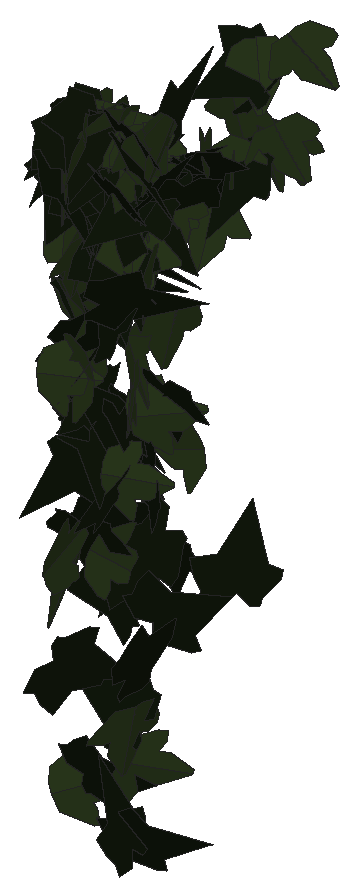
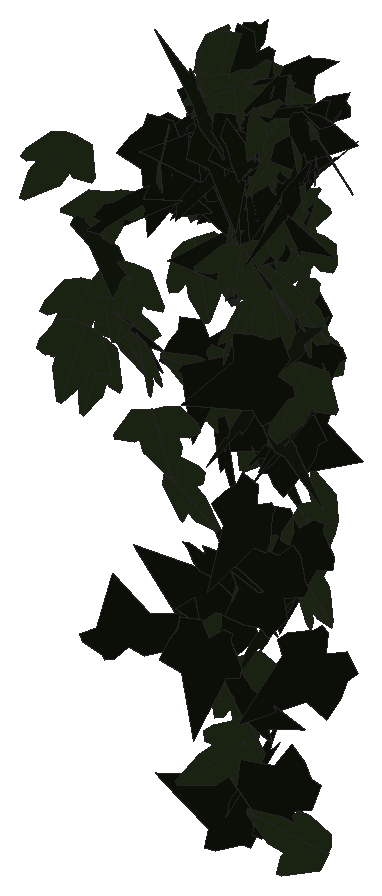
# SketchUp Ruby script. Lengths in inches.
U = 1.inch
M = Sketchup.active_model
def pt(a) = Geom::Point3d.new(a.map { |v| v * U })
def face(e, loops, mat)
  f = e.add_face(loops[0].map { |a| pt(a) })
  loops[1..].each { |l| e.add_face(l.map { |a| pt(a) }).erase! }
  f.material = f.back_material = mat if mat
  f
end
# faces: each face lists its corners as indices into pts; further lists are holes
def faces(e, pts, list, mat = nil) = list.each { |f| face(e, (f[0].is_a?(Array) ? f : [f]).map { |l| l.map { |i| pts[i] } }, mat) }
# xy, xz, yz: faces in a plane at the given z, y or x. An outline is a flat list of corners, or four numbers for a rectangle; further outlines are holes
def ring(l) = l.size == 4 ? [[l[0], l[1]], [l[2], l[1]], [l[2], l[3]], [l[0], l[3]]] : l.each_slice(2).to_a
def flat(e, list, mat, &to3) = list.each { |f| face(e, (f[0].is_a?(Array) ? f : [f]).map { |l| ring(l).map { |u, v| to3.(u, v) } }, mat) }
def xy(e, z, list, mat = nil) = flat(e, list, mat) { |x, y| [x, y, z] }
def xz(e, y, list, mat = nil) = flat(e, list, mat) { |x, z| [x, y, z] }
def yz(e, x, list, mat = nil) = flat(e, list, mat) { |y, z| [x, y, z] }
def lines(e, pts, list) = list.each { |a, b| e.add_line(pt(pts[a]), pt(pts[b])) }
# prism: a flat outline (further loops are holes) pulled along v
def prism(e, loops, v, mat = nil)
  f = face(e, loops, mat); d = Geom::Vector3d.new(v.map { |x| x * U })
  f.pushpull(f.normal.samedirection?(d) ? d.length : -d.length)
end
def box(e, o, s, mat = nil) = prism(e, [[o, [o[0] + s[0], o[1], o[2]], [o[0] + s[0], o[1] + s[1], o[2]], [o[0], o[1] + s[1], o[2]]]], [0, 0, s[2]], mat)
def at(x, y, z, deg = 0) = Geom::Transformation.translation(pt([x, y, z])) * Geom::Transformation.rotation(ORIGIN, Z_AXIS, deg.degrees)
def axes(o, x, y, z) = Geom::Transformation.new([*x, 0, *y, 0, *z, 0, *pt(o).to_a, 1])
def part(name) = M.definitions.add(name)
# library, detail: a bought-in or finely detailed component or shape, given as its bounding box
def library(name, o, s) = part(name).tap { |d| box(d.entities, o, s) }
def detail(e, o, s) = box(e.add_group.entities, o, s)
def put(e, d, t, mat = nil) = e.add_instance(d, t).tap { |i| i.material = mat if mat }
def group(e, t, mat = nil) = e.add_group.tap { |g| g.transformation = t; g.material = mat if mat }.entities
root = M.entities
M.materials.add("efeu1").color = [18, 25, 13]
M.materials.add("efeu2").color = [43, 57, 29]
c1 = part("ivyleaf_9")
p = [[1.54,2.16,1.25],[1.36,2.04,1.19],[-0.21,0.99,0.68],[-0.71,1.11,0.82],[-0.85,0.86,0.67],[-0.8,0.17,0.21],
  [-0.9,-0.01,0.1],[-0.67,-0.16,-0.02],[-0.08,-0.08,-0.05],[-0.03,-0.6,-0.4],[0.65,-0.88,-0.66],[0.83,-0.6,-0.49],
  [1.29,-0.42,-0.43],[1.8125,-0.07,-0.26],[1.21,0.44,0.15]]
faces(c1.entities,p,[[0,1,2,3,4,5,6,7,8,9,10,11,12,13,14]],"efeu1")
c2 = part("ivyleaf_10")
p = [[0,0.5,-0.03],[-0.0625,2.02,-0.43],[-0.19,2.01,-0.46],[-0.54,1.05,-0.29],[-0.52,0.625,-0.18],[-0.83,0.76,-0.28],
  [-1.16,0.64,-0.33],[-1.15,0.33,-0.24],[-0.77,-0.39,0.02],[-0.3,-0.51,0.16],[0.04,-0.48,0.23],[-0.02,2.01,-0.4375],
  [-0.06,2.01,-0.43],[0.04,-0.49,0.23],[0.67,-0.49,0.14],[1.38,0.36,-0.2],[1.375,0.51,-0.24],[0.81,0.65,-0.19],
  [0.62,0.59,-0.15],[0.6,1.09,-0.28],[0.5,1.23,-0.31]]
faces(c2.entities,p,[[0,1,2,3,4,5,6,7,8,9,10],[11,12,0,13,14,15,16,17,18,19,20]],"efeu2")
put(root,c1,axes([545.61,136.74,199.4],[0.63239,0.17677,0.4577],[0.42669,0.17049,-0.65539],[-0.24223,0.7618,0.04047]))
put(root,c2,axes([546.11,140.69,199.7],[0.68213,0.44243,-0.14411],[-0.17077,0.00015,-0.80787],[-0.43284,0.69719,0.09162]))
put(root,c1,axes([546.1,134.98,203.92],[0.41864,-0.09963,-0.78482],[-0.51595,0.63873,-0.3563],[0.59972,0.61905,0.24132]))
put(root,c2,axes([546.69,134.25,199.875],[0.06447,0.00912,-0.85901],[-0.63743,0.57799,-0.0417],[0.5759,0.63873,0.05001]))
put(root,c2,axes([546.13,134.99,198.29],[-0.41829,-0.63523,-0.40609],[0.26002,0.31436,-0.75958],[0.70768,-0.49097,0.03906]))
put(root,c2,axes([546.22,135.08,204.94],[0.42247,-0.7153,-0.04041],[0.04281,0.07203,-0.82749],[0.71516,0.41824,0.0734]))
put(root,c1,axes([545.76,135.46,199.64],[0.53861,-0.60321,-0.07073],[0.1239,0.20168,-0.77649],[0.59457,0.50441,0.22588]))
put(root,c1,axes([546.33,135.1,205.17],[0.02686,-0.08138,-0.82508],[0.27504,-0.77789,0.08568],[-0.78214,-0.27634,0.0018]))
put(root,c1,axes([546.68,134.18,205.14],[-0.76345,0.21406,-0.26205],[0.25896,-0.04664,-0.79254],[-0.21779,-0.80582,-0.02374]))
put(root,c1,axes([546.89,135.11,196.85],[-0.59699,0.5547,0.02639],[-0.02109,0.01607,-0.81491],[-0.55492,-0.59736,0.00258]))
put(root,c1,axes([547.1875,134.78,202.4],[-0.38586,0.27044,0.67565],[-0.52247,0.42944,-0.47026],[-0.50664,-0.64883,-0.02962]))
put(root,c2,axes([546.625,135.43,200.49],[-0.11591,-0.80635,0.00121],[0.0201,-0.00411,-0.81438],[0.8061,-0.11584,0.02048]))
put(root,c2,axes([546.48,135.21,205.03],[0.02633,-0.46906,-0.67824],[0.19734,0.66245,-0.45048],[0.80067,-0.14785,0.13334]))
put(root,c2,axes([546.66,135.04,202.78],[-0.10519,-0.61205,0.52001],[0.05814,-0.52888,-0.61073],[0.80103,-0.04199,0.11261]))
put(root,c1,axes([546.4,134.43,203.5625],[-0.20295,-0.72127,0.44661],[0.10126,-0.47653,-0.72356],[0.84228,-0.1165,0.1946]))
put(root,c2,axes([546.58,134.14,192.11],[0.23697,-0.69809,0.4273],[0.16665,-0.39438,-0.73672],[0.80134,0.28845,0.02686]))
put(root,c2,axes([546.32,134.5,201.97],[0.64893,0.30322,0.3824],[0.30225,0.24981,-0.711],[-0.38316,0.71059,0.08678]))
put(root,c1,axes([546.46,133.89,198.91],[0.4772,0.52153,0.62438],[0.41266,0.46866,-0.70685],[-0.70111,0.63082,0.00894]))
put(root,c2,axes([546.17,134.57,185.02],[0.32928,0.01072,-0.79971],[0.79309,0.10729,0.32799],[0.10327,-0.85817,0.03102]))
put(root,c1,axes([546.23,135.67,192.52],[0.70579,0.31997,-0.30043],[0.21253,0.24863,0.76407],[0.38402,-0.72566,0.12931]))
put(root,c1,axes([546.9,134.19,193.42],[0.65453,0.36972,-0.41326],[-0.35074,-0.21914,-0.75156],[-0.42949,0.74241,-0.01604]))
put(root,c1,axes([546.54,135.07,196.45],[0.17609,-0.79948,0.16462],[0.02458,-0.16314,-0.81857],[0.81588,0.17746,-0.01087]))
put(root,c1,axes([546.71,136.125,195.03],[0.77795,0.04309,-0.26893],[-0.26975,0.00954,-0.77879],[-0.0376,0.82306,0.0231]))
put(root,c2,axes([546.71,140.51,201.54],[0.67204,-0.44105,0.22768],[0.20511,-0.10222,-0.80342],[0.45199,0.70216,0.02606]))
put(root,c1,axes([546.89,135.14,205.49],[-0.53508,-0.61574,-0.12557],[0.09523,0.08357,-0.81557],[0.62115,-0.54323,0.01686]))
put(root,c2,axes([546.74,133.73,204.45],[-0.41519,0.41173,-0.57655],[0.18834,-0.58007,-0.54987],[-0.68298,-0.41026,0.19885]))
put(root,c2,axes([547.03,135.24,205.375],[-0.06291,-0.81765,-0.05684],[-0.01553,0.05818,-0.81982],[0.81947,-0.06167,-0.0199]))
put(root,c1,axes([546.61,134.11,205.38],[0.03815,-0.75855,-0.42726],[0.08293,0.42889,-0.75404],[0.86664,-0.00765,0.09097]))
put(root,c2,axes([546.86,135.02,205.39],[0.76183,0.29375,-0.05461],[-0.04328,-0.03951,-0.81622],[-0.29563,0.76276,-0.02125]))
put(root,c2,axes([546.89,135.35,200.86],[-0.19322,-0.5596,-0.56445],[0.22203,0.51977,-0.5913],[0.76319,-0.29289,0.02912]))
put(root,c2,axes([546.98,141.9,201.81],[-0.80811,0.1931,-0.06685],[0.06148,-0.03029,-0.83072],[-0.19487,-0.8103,0.01512]))
put(root,c1,axes([546.8,133.32,189.59],[0.02204,0.08481,-0.91651],[-0.16467,0.90235,0.07954],[0.90558,0.16201,0.03677]))
put(root,c2,axes([547.07,140.625,203.3],[-0.80095,-0.1323,-0.04872],[0.05105,-0.01019,-0.81159],[0.13142,-0.80236,0.01834]))
put(root,c2,axes([547.6,133.39,198.49],[0.21564,-0.19118,-0.90246],[-0.69715,0.57316,-0.288],[0.60412,0.72967,-0.01023]))
put(root,c1,axes([546.6,133.5,204.46],[0.50245,-0.71675,-0.00209],[-0.00204,0.00112,-0.87532],[0.71675,0.50246,-0.00103]))
put(root,c1,axes([547.08,134.77,204.45],[0.6357,0.37801,-0.34333],[-0.35969,-0.05768,-0.72951],[-0.36248,0.72019,0.12178]))
put(root,c1,axes([547.21,134.02,195.8125],[-0.02693,-0.00723,-0.85682],[0.23533,-0.82434,-0.00044],[-0.8239,-0.23522,0.02788]))
put(root,c1,axes([547.18,137.35,191.61],[0.63912,0.27311,-0.45217],[-0.40769,-0.1963,-0.69482],[-0.33591,0.75789,-0.01703]))
put(root,c2,axes([547.2,133.8,202.13],[0.06647,-0.85038,-0.03459],[0.00194,0.03485,-0.85296],[0.85108,0.06633,0.00464]))
put(root,c2,axes([547.24,132.76,192.94],[0.16811,-0.30744,0.92992],[-0.32559,0.87232,0.34726],[-0.92372,-0.36342,0.04684]))
put(root,c1,axes([546.94,135.54,190.92],[0.54706,-0.68574,-0.42646],[0.26362,-0.33523,0.87721],[-0.76329,-0.60726,-0.00268]))
put(root,c1,axes([547.55,135.07,201.36],[-0.71082,0.40271,-0.09212],[0.08434,-0.03801,-0.81693],[-0.40441,-0.71576,-0.00845]))
put(root,c2,axes([546.58,133.37,198.25],[0.13669,-0.19673,-0.77637],[0.78336,-0.1311,0.17114],[-0.16671,-0.77733,0.16762]))
put(root,c1,axes([546.97,134.5,203.62],[0.04386,-0.85651,-0.16835],[-0.02143,0.16746,-0.85754],[0.87263,0.04716,-0.0126]))
put(root,c1,axes([547.4375,133.27,198.36],[0.12962,0.51972,0.62303],[-0.01566,0.63241,-0.52429],[-0.81119,0.07084,0.10967]))
put(root,c1,axes([547.03,134.62,196.34],[0.07655,-0.80206,0.06377],[0.02846,-0.06132,-0.8054],[0.80409,0.07853,0.02243]))
put(root,c2,axes([547.48,140.42,201.96],[0.78404,-0.04348,-0.28572],[-0.28551,0.01153,-0.78524],[0.0448,0.8344,-0.00403]))
put(root,c1,axes([546.85,134.44,196.92],[-0.12305,-0.06856,-0.87052],[0.68325,0.53988,-0.1391],[0.54377,-0.69388,-0.02221]))
put(root,c2,axes([547.48,134.78,204.21],[0.04292,-0.81362,0.15034],[0.00143,-0.15047,-0.81472],[0.82739,0.04247,-0.00639]))
put(root,c1,axes([547.07,134.44,204.04],[0.36162,-0.55029,-0.57723],[-0.09742,0.59857,-0.63166],[0.79153,0.32508,0.18597]))
put(root,c2,axes([547.27,135.95,201.91],[0.40906,0.69555,0.05472],[0.02898,0.04644,-0.80692],[-0.69709,0.41008,-0.00143]))
put(root,c1,axes([547.5,134.75,204.91],[-0.39146,-0.6806,0.22902],[-0.12295,-0.19347,-0.78509],[0.7075,-0.4102,-0.00971]))
put(root,c1,axes([547.89,140.57,204.09],[-0.07567,0.62355,0.52426],[-0.27553,0.47589,-0.60579],[-0.76664,-0.23258,0.16598]))
put(root,c1,axes([547.6,140.49,201.95],[-0.77482,-0.18215,-0.25497],[0.27034,-0.04472,-0.78959],[0.15844,-0.81447,0.10037]))
put(root,c1,axes([546.9,134.83,202.18],[0.22154,-0.01211,0.8427],[0.82646,0.17379,-0.21478],[-0.16508,0.85383,0.05566]))
put(root,c2,axes([547.56,133.4,205.55],[0.21084,-0.7276,-0.46431],[-0.00285,0.47738,-0.74936],[0.86312,0.17931,0.11094]))
put(root,c2,axes([547.52,142.05,202.07],[-0.82513,-0.071,-0.10658],[0.10721,-0.00285,-0.82809],[0.07005,-0.83198,0.01193]))
put(root,c1,axes([547.6,135.31,204.32],[0.33624,0.21352,0.71521],[-0.59527,-0.39652,0.39823],[0.45028,-0.68363,-0.0076]))
put(root,c1,axes([547.72,140.73,204.82],[-0.42701,-0.41233,0.56307],[-0.31397,-0.47604,-0.5867],[0.62329,-0.52228,0.09022]))
put(root,c2,axes([547.3125,135.17,200.45],[0.78736,-0.09526,0.19053],[0.18664,-0.04317,-0.79286],[0.10268,0.80894,-0.01987]))
put(root,c1,axes([547.5,134.11,206],[-0.33067,-0.77131,0.05423],[-0.01346,-0.05323,-0.83916],[0.77309,-0.33083,0.00859]))
put(root,c2,axes([547.49,134.37,192.5625],[0.06112,0.52183,0.68495],[0.00049,0.68665,-0.52317],[-0.86108,0.03744,0.04832]))
put(root,c1,axes([546.91,134.43,185.76],[0.26983,-0.16319,0.8108],[0.71268,-0.38687,-0.31505],[0.41965,0.76193,0.01369]))
put(root,c1,axes([547.875,135.19,204.97],[-0.48149,0.44735,-0.49059],[0.2867,-0.4065,-0.65207],[-0.59883,-0.55431,0.08227]))
put(root,c2,axes([547.84,134.59,205.82],[-0.11987,-0.82428,0.1953],[-0.05748,-0.18887,-0.83245],[0.84515,-0.12975,-0.02892]))
put(root,c2,axes([548.29,136.02,190.43],[-0.20039,0.20317,-0.7828],[-0.61998,0.47927,0.2831],[0.51931,0.65057,0.03591]))
put(root,c2,axes([547.85,135.23,201.97],[0.09469,-0.76625,-0.28768],[0.00917,0.29058,-0.77094],[0.81842,0.0854,0.04192]))
put(root,c2,axes([547.35,135.35,203.32],[0.10686,-0.09981,0.80268],[0.68224,-0.42383,-0.14352],[0.43453,0.68999,0.02795]))
put(root,c2,axes([547.84,135.21,201.83],[-0.24546,0.78445,0.04881],[-0.0027,0.05029,-0.82187],[-0.78596,-0.24516,-0.01242]))
put(root,c2,axes([547.78,140.51,205.2],[0.56827,0.58383,0.07739],[0.05556,0.05393,-0.81473],[-0.58631,0.57097,-0.00219]))
put(root,c1,axes([548.3125,135.86,192.92],[-0.97657,-0.05472,-0.15829],[0.15803,0.00906,-0.9781],[0.05547,-0.98928,-0.00021]))
put(root,c1,axes([548.73,134.24,188.14],[-0.34865,0.2625,0.75661],[-0.60627,0.45266,-0.43642],[-0.52327,-0.69937,0.00152]))
put(root,c1,axes([548.35,135.25,204.51],[-0.133,0.81127,0.00535],[-0.00568,0.00449,-0.82208],[-0.81127,-0.13303,0.00488]))
put(root,c1,axes([547.78,134.56,197.13],[0.61895,-0.39521,-0.35068],[-0.24125,0.26914,-0.72913],[0.47007,0.65852,0.08754]))
put(root,c1,axes([547.4375,135.27,201.5],[0.65204,-0.24081,0.43804],[0.44754,-0.03946,-0.68788],[0.22266,0.78453,0.09986]))
put(root,c2,axes([548.1,134.84,205.54],[0.52459,0.6027,-0.26902],[-0.17902,-0.20082,-0.79902],[-0.63527,0.55429,0.00302]))
put(root,c1,axes([548.56,133.57,195.33],[-0.61045,0.56333,-0.07607],[0.05617,-0.05129,-0.83065],[-0.56566,-0.61303,-0.0004]))
put(root,c2,axes([548.71,136.6,195.28],[0.33121,-0.14022,-0.75629],[-0.67444,0.34297,-0.35895],[0.36983,0.75104,0.02271]))
put(root,c1,axes([548.06,134.34,203.26],[0.45689,0.44228,0.51735],[0.28828,0.43871,-0.62964],[-0.61657,0.53286,0.08898]))
put(root,c2,axes([548.15,141.04,202.65],[-0.46181,-0.62071,-0.33517],[0.3329,0.16142,-0.75763],[0.62193,-0.54731,0.15666]))
put(root,c1,axes([547.73,134.29,201.73],[0.31058,-0.53856,0.66865],[0.53052,-0.43869,-0.59975],[0.67505,0.59254,0.16371]))
put(root,c1,axes([548.42,134.42,202.39],[-0.29731,-0.57673,0.50695],[-0.06399,-0.52312,-0.63265],[0.76519,-0.26783,0.14406]))
put(root,c1,axes([549.04,134.79,203.65],[-0.37806,0.79541,0.46608],[-0.18486,0.42811,-0.88056],[-0.90318,-0.42058,-0.01487]))
put(root,c1,axes([548.44,135.27,204.59],[0.68503,0.42401,-0.16594],[-0.22759,0.05921,-0.78822],[-0.39437,0.70235,0.16663]))
put(root,c1,axes([549.04,133.05,200.46],[-0.25009,0.51858,0.59693],[-0.27243,0.53123,-0.57564],[-0.74231,-0.36968,0.01015]))
put(root,c2,axes([548.52,134.4,199.19],[-0.32648,0.79351,0.09053],[-0.04173,0.08072,-0.85801],[-0.79757,-0.32905,0.00783]))
put(root,c2,axes([548.48,134.6,205.35],[0.48386,0.66196,-0.08873],[-0.07735,-0.05329,-0.81936],[-0.66338,0.48903,0.03082]))
put(root,c1,axes([548.32,133.89,202.45],[-0.48763,-0.47094,-0.5863],[0.46477,0.36061,-0.67621],[0.5912,-0.67193,0.04801]))
put(root,c1,axes([548.48,133.32,204.64],[0.7687,0.05488,-0.39208],[-0.39453,0.03492,-0.76862],[-0.03295,0.86221,0.05609]))
put(root,c1,axes([548.53,133.87,206.12],[0.76119,0.06902,-0.43395],[-0.43534,0.00065,-0.76352],[-0.05964,0.87619,0.03475]))
put(root,c1,axes([548.16,135.17,203.95],[0.45127,0.02852,0.69238],[0.54453,0.49644,-0.37535],[-0.4286,0.66074,0.25213]))
put(root,c1,axes([548.48,134.43,202.43],[-0.08708,-0.79484,-0.19801],[0.0466,0.194,-0.79922],[0.8178,-0.09569,0.02446]))
put(root,c1,axes([548.51,135.65,205.15],[-0.34456,0.83228,0.41351],[0.15556,-0.38314,0.90078],[0.91623,0.37804,0.00256]))
put(root,c1,axes([549.28,134.27,195.73],[0.08048,-0.02272,-0.87671],[-0.87219,0.09002,-0.0824],[0.09174,0.87578,-0.01427]))
put(root,c2,axes([548.73,134.53,205.55],[0.48299,0.66852,-0.04524],[-0.05469,-0.01624,-0.82401],[-0.66781,0.48483,0.03477]))
put(root,c2,axes([548.96,133.76,188.45],[-0.22381,-0.92534,0.01728],[-0.00037,-0.01769,-0.95202],[0.9255,-0.22378,0.0038]))
put(root,c1,axes([549.0625,134.53,204.01],[-0.68359,-0.41977,0.28887],[-0.07473,-0.39553,-0.75161],[0.50405,-0.62793,0.28033]))
put(root,c1,axes([548.75,135.2,204.89],[-0.17927,-0.80186,0.04268],[-0.01045,-0.0414,-0.82165],[0.80293,-0.17957,-0.00116]))
put(root,c2,axes([548.82,134.07,204.48],[0.33807,0.57935,0.48627],[-0.01212,0.53671,-0.63102],[-0.75628,0.25038,0.22748]))
put(root,c2,axes([548.65,134.24,186.83],[-0.24177,-0.28773,-0.79689],[0.54129,0.58507,-0.37547],[0.65179,-0.59261,0.01623]))
put(root,c2,axes([548.34,133.95,195.52],[0.08744,-0.13092,-0.85883],[0.85752,-0.12532,0.10641],[-0.13922,-0.85412,0.11603]))
put(root,c1,axes([549.28,133.31,184.92],[-0.12489,-0.72973,0.45929],[0.08146,0.45202,0.74033],[-0.85838,0.14907,0.00343]))
put(root,c2,axes([548.92,133.83,202.63],[0.6356,0.67014,-0.01474],[-0.01954,-0.00178,-0.92353],[-0.67002,0.63577,0.01295]))
put(root,c2,axes([549.42,136.3125,204.09],[-0.03024,0.09779,-0.81771],[-0.29825,0.76141,0.10209],[0.76763,0.29969,0.00745]))
put(root,c1,axes([548.8125,134.32,203.47],[0.22715,-0.47507,-0.6384],[-0.05462,0.65303,-0.50539],[0.79389,0.18085,0.14789]))
put(root,c2,axes([548.88,133.97,198.45],[-0.23849,0.26662,-0.79049],[0.25878,-0.75796,-0.33372],[-0.7931,-0.32749,0.12882]))
put(root,c2,axes([549.08,135.0625,203.34],[0.16326,0.76137,-0.29058],[-0.05222,-0.28597,-0.77864],[-0.81327,0.17121,-0.00833]))
put(root,c1,axes([549.18,136.04,204.39],[0.54033,0.60153,-0.1539],[-0.15387,-0.06792,-0.80572],[-0.60154,0.5577,0.06786]))
put(root,c2,axes([549.0625,135.07,203.41],[0.11914,0.81646,0.10287],[0.0043,0.10332,-0.82504],[-0.8229,0.11875,0.01058]))
put(root,c1,axes([549.27,134.74,198.17],[0.65146,0.26325,-0.48071],[-0.44883,-0.17226,-0.7026],[-0.31452,0.79108,0.00697]))
put(root,c2,axes([549.2,135.04,203.61],[-0.67041,-0.48248,-0.10161],[0.17938,-0.07893,-0.8088],[0.45928,-0.67346,0.16758]))
put(root,c2,axes([549.26,133.97,206.08],[-0.24449,-0.75401,-0.33591],[0.17269,0.29586,-0.7898],[0.80718,-0.29168,0.06722]))
put(root,c1,axes([549.3125,134.13,204.25],[0.23084,0.59351,0.53115],[0.14705,0.51174,-0.63574],[-0.78278,0.27116,0.03721]))
put(root,c1,axes([549.18,133.33,190.01],[0.14199,0.11651,0.91878],[0.46498,0.7949,-0.17266],[-0.80095,0.48212,0.06264]))
put(root,c2,axes([548.67,134.6875,197.17],[0.20404,0.04589,-0.87023],[0.8686,0.06139,0.2069],[0.0703,-0.89172,-0.03054]))
put(root,c1,axes([548.88,133.6,205.75],[0.67202,-0.53776,0.07978],[0.05973,-0.05305,-0.86068],[0.54035,0.67466,-0.00408]))
put(root,c2,axes([549.26,134.28,202.25],[0.44409,-0.66404,0.31124],[0.23807,-0.21361,-0.79544],[0.69364,0.49845,0.07375]))
put(root,c1,axes([549.73,134.97,204.21],[0.02943,0.63866,-0.53812],[-0.11652,-0.53005,-0.63545],[-0.82698,0.09741,0.07038]))
put(root,c1,axes([549.47,137.58,190.89],[-0.59069,-0.2827,0.53435],[0.53229,0.11091,0.6471],[-0.28656,0.78876,0.10053]))
put(root,c1,axes([548.87,134.95,190.84],[0.02088,-0.0106,0.88885],[0.84768,-0.26741,-0.0231],[0.26759,0.84793,0.00382]))
put(root,c2,axes([549.65,134.67,200.47],[-0.33202,-0.78691,0.08326],[-0.03039,-0.07755,-0.85409],[0.79072,-0.3334,0.00213]))
put(root,c1,axes([548.79,133.79,184.64],[0.33807,-0.16051,0.79315],[0.78874,-0.12685,-0.36186],[0.18095,0.85281,0.09545]))
put(root,c2,axes([549.28,140.37,206.09],[-0.41245,-0.55293,-0.4565],[0.48698,0.17052,-0.64654],[0.52628,-0.59112,0.2405]))
put(root,c2,axes([549.43,134.58,205.94],[0.19821,-0.60512,0.54647],[0.2342,-0.49643,-0.63466],[0.78099,0.30244,0.05163]))
put(root,c1,axes([548.99,132.57,201.54],[0.58978,0.22043,0.72035],[0.66324,0.28189,-0.62928],[-0.35722,0.88729,0.02096]))
